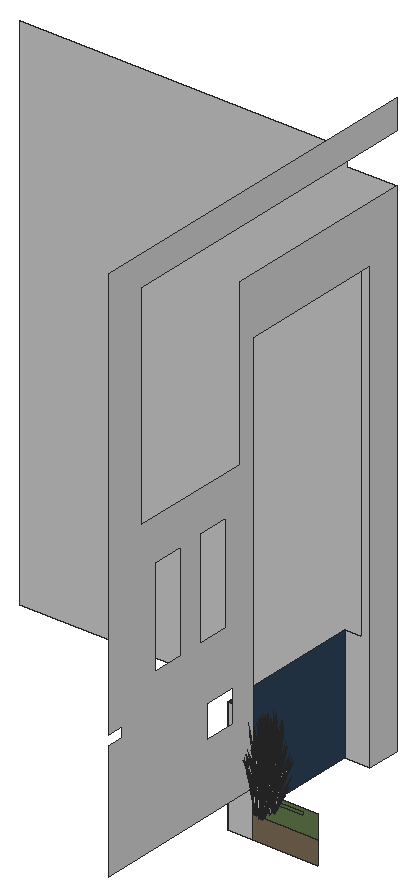
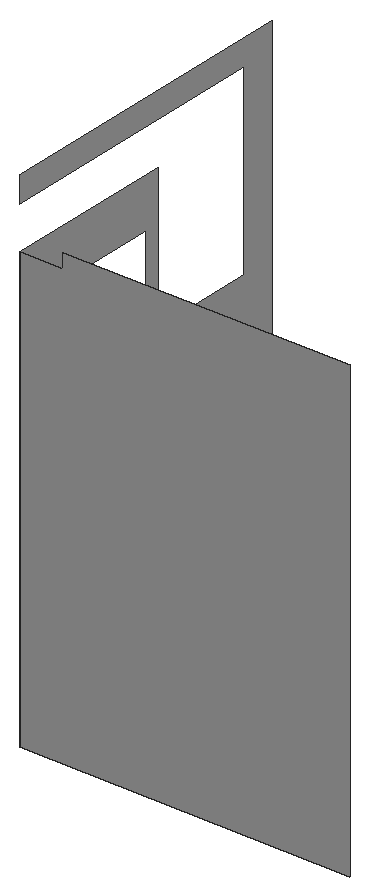
# SketchUp Ruby script. Lengths in inches.
U = 1.inch
M = Sketchup.active_model
def pt(a) = Geom::Point3d.new(a.map { |v| v * U })
def face(e, loops, mat)
  f = e.add_face(loops[0].map { |a| pt(a) })
  loops[1..].each { |l| e.add_face(l.map { |a| pt(a) }).erase! }
  f.material = f.back_material = mat if mat
  f
end
# faces: each face lists its corners as indices into pts; further lists are holes
def faces(e, pts, list, mat = nil) = list.each { |f| face(e, (f[0].is_a?(Array) ? f : [f]).map { |l| l.map { |i| pts[i] } }, mat) }
# xy, xz, yz: faces in a plane at the given z, y or x. An outline is a flat list of corners, or four numbers for a rectangle; further outlines are holes
def ring(l) = l.size == 4 ? [[l[0], l[1]], [l[2], l[1]], [l[2], l[3]], [l[0], l[3]]] : l.each_slice(2).to_a
def flat(e, list, mat, &to3) = list.each { |f| face(e, (f[0].is_a?(Array) ? f : [f]).map { |l| ring(l).map { |u, v| to3.(u, v) } }, mat) }
def xy(e, z, list, mat = nil) = flat(e, list, mat) { |x, y| [x, y, z] }
def xz(e, y, list, mat = nil) = flat(e, list, mat) { |x, z| [x, y, z] }
def yz(e, x, list, mat = nil) = flat(e, list, mat) { |y, z| [x, y, z] }
def lines(e, pts, list) = list.each { |a, b| e.add_line(pt(pts[a]), pt(pts[b])) }
# prism: a flat outline (further loops are holes) pulled along v
def prism(e, loops, v, mat = nil)
  f = face(e, loops, mat); d = Geom::Vector3d.new(v.map { |x| x * U })
  f.pushpull(f.normal.samedirection?(d) ? d.length : -d.length)
end
def box(e, o, s, mat = nil) = prism(e, [[o, [o[0] + s[0], o[1], o[2]], [o[0] + s[0], o[1] + s[1], o[2]], [o[0], o[1] + s[1], o[2]]]], [0, 0, s[2]], mat)
def at(x, y, z, deg = 0) = Geom::Transformation.translation(pt([x, y, z])) * Geom::Transformation.rotation(ORIGIN, Z_AXIS, deg.degrees)
def axes(o, x, y, z) = Geom::Transformation.new([*x, 0, *y, 0, *z, 0, *pt(o).to_a, 1])
def part(name) = M.definitions.add(name)
# library, detail: a bought-in or finely detailed component or shape, given as its bounding box
def library(name, o, s) = part(name).tap { |d| box(d.entities, o, s) }
def detail(e, o, s) = box(e.add_group.entities, o, s)
def put(e, d, t, mat = nil) = e.add_instance(d, t).tap { |i| i.material = mat if mat }
def group(e, t, mat = nil) = e.add_group.tap { |g| g.transformation = t; g.material = mat if mat }.entities
root = M.entities
M.materials.add("Carpet_04_1K").color = [43, 65, 85]
M.materials.add("LightPink_Translucent").color = [144, 107, 117]
M.materials["LightPink_Translucent"].alpha = 0.75
M.materials.add("Plaster_03_1K").color = [121, 105, 83]
M.materials.add("Roofing_02_1K").color = [97, 118, 74]
M.materials.add("[_0053_Ivory_]").color = [200, 200, 200]
c1 = part("blade")
p = [[2.15,0.21,22],[0,0.17,0],[0.09,0.45,0],[2.18,0.31,22],[2.29,0.31,22],[0.38,0.45,0],
  [2.48,0.24,33],[2.49,0.24,33],[2.48,0.22,33]]
faces(c1.entities,p,[[0,1,2,3],[4,5,2,3],[6,3,4,7],[8,0,3,6]])
c2 = part("seeds")
p = [[0.3,-0.1,1.38],[-0.01,-0.03,1.59],[-0.01,-0.03,0.03],[0.14,-0.07,-0.07],[0.29,-0.03,3],[0.15,0.01,3.11]]
faces(c2.entities,p,[[0,1,2,3],[1,0,4,5]],"LightPink_Translucent")
c3 = part("blade with seeds")
put(c3.entities,c1,at(0,0,0))
put(c3.entities,c2,axes([2.4,0.25,30.99],[1.5799,-0.05474,1.17369],[-0.12525,1.92788,0.29478],[-0.07173,-0.02425,1.56792]))
xz(root,365.15,[[659.51,34,695.51,36]],"Roofing_02_1K")
xz(root,371.15,[[653.51,0,701.51,17]],"Plaster_03_1K")
xz(root,371.15,[[653.51,17,701.51,34]],"Roofing_02_1K")
xz(root,371.15,[[635.1,0,653.51,84]],"[_0053_Ivory_]")
xz(root,479.15,[[635.1,0,653.51,0,653.51,330,647.1,330,647.1,84,635.1,84]],"[_0053_Ivory_]")
xz(root,503.15,[[377.51,0,377.51,384,617.51,384,617.51,372,653.51,372,653.51,0]],"[_0053_Ivory_]")
yz(root,635.1,[[371.15,0,479.15,84]],"Carpet_04_1K")
yz(root,653.51,[[[479.15,0,503.15,0,503.15,372,359.15,372,359.15,252,269.15,252,269.15,408,503.15,408,503.15,430,239.15,430,239.15,127,251.15,127,251.15,120,239.15,120,239.15,34,371.15,34,371.15,84,329.15,84,329.15,108,353.15,108,353.15,84,371.15,84,371.15,330,479.15,330],[323.15,150,347.15,222],[281.15,150,305.15,222]]],"[_0053_Ivory_]")
put(root,c3,axes([677.21,343.38,38.33],[-0.16454,0.57202,-0.51099],[-0.56413,-0.19607,-0.3958],[-0.22713,0.05245,0.97773]),"[_0053_Ivory_]")
put(root,c3,axes([680.74,343.13,35.86],[0.36485,0.52782,-0.44739],[-0.55265,0.37168,0.21531],[0.11807,0.06531,1.43643]),"[_0053_Ivory_]")
put(root,c3,axes([683.21,345.36,37.58],[-0.11624,-0.52862,-0.03492],[0.54943,-0.12153,-0.15832],[0.11473,0.03351,0.52218]),"[_0053_Ivory_]")
put(root,c3,axes([678.47,345.83,36.03],[-0.37973,0.63014,0],[-0.6353,-0.35142,-0.51607],[-0.14469,-0.08004,1.63711]),"[_0053_Ivory_]")
put(root,c3,axes([682.35,343.64,36.13],[0,-0.62885,0.49651],[0.67951,0,0],[0,0.14322,1.57504]),"[_0053_Ivory_]")
put(root,c3,axes([680.65,344.11,36.37],[0.65953,-0.03882,0.44739],[0.05964,0.64439,-0.21531],[-0.11807,0.06531,1.43643]),"[_0053_Ivory_]")
put(root,c3,axes([681.06,343.45,36.27],[0.56587,-0.18339,0.1448],[0.19817,0.52368,-0.41347],[0,0.11525,1.26744]),"[_0053_Ivory_]")
put(root,c3,axes([680.06,344.42,35.86],[-0.65953,0.03882,-0.44739],[-0.05964,-0.64439,0.21531],[-0.11807,0.06531,1.43643]),"[_0053_Ivory_]")
put(root,c3,axes([683.16,344.73,36.24],[-0.14627,-0.15466,1.43002],[0.19032,-0.51164,-0.30754],[0.29594,0.06931,0.61141]),"[_0053_Ivory_]")
put(root,c3,axes([680.55,345.29,35.86],[0.61229,0.28233,0],[-0.29468,0.58663,0],[0,0,1.74954]),"[_0053_Ivory_]")
put(root,c3,axes([680.79,345.92,35.85],[-0.37499,-0.63235,-0.05142],[0.6353,-0.35142,0.51607],[-0.15655,0.0602,1.6363]),"[_0053_Ivory_]")
put(root,c3,axes([680.66,344.39,36.27],[0.44871,0.37783,0.1448],[-0.37428,0.42627,-0.41347],[-0.10418,0.05763,1.26744]),"[_0053_Ivory_]")
put(root,c3,axes([677.1875,343.68,37.53],[0.21074,-0.13302,1.71376],[0.17741,0.61464,0.13857],[-0.33083,0.13891,0.73262]),"[_0053_Ivory_]")
put(root,c3,axes([678.49,351.64,37.53],[0.13883,0.2019,1.71376],[-0.64153,0.16998,0.13857],[-0.14499,-0.31697,0.73262]),"[_0053_Ivory_]")
put(root,c3,axes([681.82,345.04,38.63],[0.60713,0.01514,-0.71045],[-0.04078,0.63759,0.08574],[0.25721,0.06729,1.00501]),"[_0053_Ivory_]")
put(root,c3,axes([680.98,351.35,36.24],[-0.17264,0.12729,1.43002],[-0.51703,-0.22279,-0.30754],[0.09584,-0.27707,0.61141]),"[_0053_Ivory_]")
put(root,c3,axes([681.13,345.55,36.13],[0.56842,-0.31443,0.49651],[0.33976,0.56381,0],[-0.12946,0.07161,1.57504]),"[_0053_Ivory_]")
put(root,c3,axes([680.2,351.79,38.63],[-0.28988,-0.51132,-0.71045],[0.59671,-0.28496,0.08574],[-0.06778,-0.24706,1.00501]),"[_0053_Ivory_]")
put(root,c3,axes([680.32,345.06,35.94],[0.26406,0.72244,-0.06012],[-0.7545,0.25315,0],[0.00922,0.02523,1.72173]),"[_0053_Ivory_]")
put(root,c3,axes([678.3125,351.11,36.24],[-0.03678,0.20572,1.43002],[-0.53767,0.17221,-0.30754],[-0.12568,-0.26589,0.61141]),"[_0053_Ivory_]")
put(root,c3,axes([680.62,345.84,35.68],[-0.56663,-0.1556,-0.30978],[0.14267,-0.54795,0.30978],[-0.11423,0.06319,1.38974]),"[_0053_Ivory_]")
put(root,c3,axes([676.53,344.73,36.24],[0.21107,0.05162,1.43002],[0.13604,0.52729,-0.30754],[-0.28671,0.0987,0.61141]),"[_0053_Ivory_]")
put(root,c3,axes([679.7,350.65,35.15],[-0.10187,0.02266,1.76342],[-0.56336,-0.25503,-0.26939],[0.00945,-0.21273,0.30037]),"[_0053_Ivory_]")
put(root,c3,axes([682.81,343.75,36.03],[0.75945,0,0],[0,0.70283,-0.51607],[0,0.16007,1.63711]),"[_0053_Ivory_]")
put(root,c3,axes([682.51,344.11,35.85],[-0.75908,-0.00503,-0.04976],[0,-0.70283,0.49943],[-0.02386,0.16,1.58352]),"[_0053_Ivory_]")
put(root,c3,axes([680.86,343.5,36.32],[0.68399,0.30005,-0.29095],[-0.32934,0.63331,-0.50002],[0.0215,0.15549,1.59708]),"[_0053_Ivory_]")
put(root,c3,axes([676.09,345.83,36.42],[0.25312,-0.28501,1.1486],[0.09988,0.45119,0.84392],[-0.18292,0.08079,0.25299]),"[_0053_Ivory_]")
put(root,c3,axes([682.18,345.3,38.18],[0.34557,0.39372,-0.35414],[-0.39459,0.37271,0.4572],[0.20048,0.05671,0.87481]),"[_0053_Ivory_]")
put(root,c3,axes([682.35,344.21,35.68],[-0.42396,0.39235,-0.30978],[-0.42396,-0.39235,0.30978],[0,0.12637,1.38974]),"[_0053_Ivory_]")
put(root,c3,axes([681.4,352.29,38.63],[0.0158,-0.58168,-0.71045],[0.66548,0.03907,0.08574],[0.07023,-0.24643,1.00501]),"[_0053_Ivory_]")
put(root,c3,axes([680.52,344.25,36.32],[0.07077,0.71755,-0.29095],[-0.73712,0.04339,-0.50002],[-0.1298,0.09558,1.59708]),"[_0053_Ivory_]")
put(root,c3,axes([680.79,343.97,35.86],[-0.29468,0.56664,-0.44739],[-0.61229,-0.27271,0.21531],[0,0.13062,1.43643]),"[_0053_Ivory_]")
put(root,c3,axes([677.04,344.6,38.18],[-0.52868,0.08987,-0.35414],[-0.1396,-0.51376,0.4572],[-0.1515,0.13799,0.87481]),"[_0053_Ivory_]")
put(root,c3,axes([680.25,351.35,38.18],[0.1831,-0.48359,-0.35414],[0.53419,0.14105,0.4572],[-0.04898,-0.1947,0.87481]),"[_0053_Ivory_]")
put(root,c3,axes([680.65,351.99,37.53],[-0.11309,0.21615,1.71376],[-0.47441,-0.44731,0.13857],[0.21402,-0.27879,0.73262]),"[_0053_Ivory_]")
put(root,c3,axes([679.98,351.6875,38.33],[-0.59704,-0.15764,-0.51099],[0.20464,-0.54049,-0.3958],[-0.05475,-0.21761,0.97773]),"[_0053_Ivory_]")
put(root,c3,axes([680.35,350.33,36.42],[0.07791,0.3667,1.1486],[-0.43222,-0.2031,0.84392],[0.04651,-0.18776,0.25299]),"[_0053_Ivory_]")
put(root,c3,axes([681.27,352.1,38.33],[-0.43478,-0.42253,-0.51099],[0.45929,-0.37004,-0.3958],[0.06615,-0.21468,0.97773]),"[_0053_Ivory_]")
put(root,c3,axes([680.08,344.8,35.71],[-0.40909,0.47266,-0.62353],[-0.50819,-0.4286,-0.16365],[-0.16393,0.11791,1.37633]),"[_0053_Ivory_]")
put(root,c3,axes([680.81,345.59,35.98],[0.76036,0.2044,0.30756],[-0.19023,0.7306,-0.36492],[-0.12585,0.09144,1.64885]),"[_0053_Ivory_]")
put(root,c3,axes([680.75,346.09,35.67],[-0.56842,0.31443,-0.49651],[-0.33976,-0.56381,0],[-0.12946,0.07161,1.57504]),"[_0053_Ivory_]")
put(root,c3,axes([682.64,344.22,35.67],[0,0.62885,-0.49651],[-0.67951,0,0],[0,0.14322,1.57504]),"[_0053_Ivory_]")
put(root,c3,axes([680.94,344.29,37.53],[-0.2256,-0.10835,1.71376],[0.46687,-0.45453,0.13857],[0.29098,0.20505,0.73262]),"[_0053_Ivory_]")
put(root,c3,axes([681.78,345.53,36.42],[-0.34197,-0.18082,1.1486],[0.44156,-0.18372,0.84392],[0.1191,0.15563,0.25299]),"[_0053_Ivory_]")
put(root,c3,axes([681.68,351.9375,38.18],[0.41095,-0.33109,-0.35414],[0.38901,0.37805,0.4572],[0.05919,-0.19208,0.87481]),"[_0053_Ivory_]")
put(root,c3,axes([678.125,350.77,36.42],[0.31682,0.21887,1.1486],[-0.4614,0.13157,0.84392],[-0.09872,-0.16821,0.25299]),"[_0053_Ivory_]")
put(root,c3,axes([678.89,351.93,38.63],[-0.51789,-0.30395,-0.71045],[0.36805,-0.53263,0.08574],[-0.18764,-0.18149,1.00501]),"[_0053_Ivory_]")
put(root,c3,axes([678.71,351.53,38.18],[-0.0938,-0.50652,-0.35414],[0.53623,-0.13375,0.4572],[-0.14403,-0.14515,0.87481]),"[_0053_Ivory_]")
put(root,c3,axes([677.96,344.09,37.53],[0.1517,-0.19322,1.71376],[0.38303,0.52154,0.13857],[-0.26271,0.23751,0.73262]),"[_0053_Ivory_]")
put(root,c3,axes([677.48,344.66,38.33],[0.15602,0.5742,-0.51099],[-0.59087,0.10045,-0.3958],[-0.16933,0.15423,0.97773]),"[_0053_Ivory_]")
put(root,c3,axes([681.27,345.99,36.03],[0.37973,0.63014,0],[-0.6353,0.35142,-0.51607],[-0.14469,0.08004,1.63711]),"[_0053_Ivory_]")
put(root,c3,axes([681.87,346.2,35.15],[0.04425,-0.09079,1.76342],[0.55709,-0.26738,-0.26939],[0.16889,0.13839,0.30037]),"[_0053_Ivory_]")
put(root,c3,axes([680.94,343.49,36.5],[-0.01659,-0.59209,1.41272],[0.75089,0.15348,0.59816],[-0.1776,0.32398,1.3335]),"[_0053_Ivory_]")
put(root,c3,axes([681.14,344.14,35.75],[0.2227,0.57576,-0.69212],[-0.64151,0.20736,-0.18165],[0.02462,0.19497,1.52773]),"[_0053_Ivory_]")
put(root,c3,axes([676.76,346.12,35.15],[0.08147,0.06283,1.76342],[0.13814,0.58211,-0.26939],[-0.18056,0.12413,0.30037]),"[_0053_Ivory_]")
put(root,c3,axes([681,345.78,38.33],[0.59932,-0.14948,-0.51099],[0.10484,0.56611,-0.3958],[0.16097,0.16223,0.97773]),"[_0053_Ivory_]")
put(root,c3,axes([677.875,351.43,35.15],[-0.05883,0.08284,1.76342],[-0.59454,0.17861,-0.26939],[-0.14363,-0.16248,0.30037]),"[_0053_Ivory_]")
put(root,c3,axes([678.86,353.71,35.75],[-0.24943,-0.64486,-0.69835],[0.71849,-0.23224,-0.18329],[-0.02757,-0.21836,1.54149]),"[_0053_Ivory_]")
put(root,c3,axes([677.56,352.27,37.53],[0.2256,0.10835,1.71376],[-0.46687,0.45453,0.13857],[-0.29098,-0.20505,0.73262]),"[_0053_Ivory_]")
put(root,c3,axes([682.19,351.74,35.15],[-0.0909,-0.04954,1.76342],[-0.2335,-0.55347,-0.26939],[0.15752,-0.1502,0.30037]),"[_0053_Ivory_]")
put(root,c3,axes([681.83,346.35,36.32],[-0.38947,-0.01972,1.0506],[0.25721,-0.41888,0.58006],[0.15386,0.14882,0.8241]),"[_0053_Ivory_]")
put(root,c3,axes([678.65,351.95,38.33],[-0.59932,0.14948,-0.51099],[-0.10484,-0.56611,-0.3958],[-0.16097,-0.16223,0.97773]),"[_0053_Ivory_]")
put(root,c3,axes([677.84,344.57,37.53],[0.11309,-0.21615,1.71376],[0.47441,0.44731,0.13857],[-0.21402,0.27879,0.73262]),"[_0053_Ivory_]")
put(root,c3,axes([682.1875,353.3,38.63],[0.31725,-0.49618,-0.71045],[0.55593,0.35263,0.08574],[0.18942,-0.17977,1.00501]),"[_0053_Ivory_]")
put(root,c3,axes([678.76,351.86,36.03],[-0.37973,-0.63014,0],[0.6353,-0.35142,-0.51607],[0.14469,-0.08004,1.63711]),"[_0053_Ivory_]")
put(root,c3,axes([682.17,353.07,38.33],[-0.15602,-0.5742,-0.51099],[0.59087,-0.10045,-0.3958],[0.16933,-0.15423,0.97773]),"[_0053_Ivory_]")
put(root,c3,axes([680.56,345.34,36.24],[0.01072,-0.20846,1.43002],[0.51218,-0.23285,-0.30754],[0.15811,0.2495,0.61141]),"[_0053_Ivory_]")
put(root,c3,axes([679.59,351.1,35.78],[-0.4197,0.36076,-0.03893],[-0.38456,-0.39511,-0.17649],[-0.02707,-0.11196,0.58215]),"[_0053_Ivory_]")
put(root,c3,axes([677.97,345.79,38.18],[-0.41095,0.33109,-0.35414],[-0.38901,-0.37805,0.4572],[-0.05919,0.19208,0.87481]),"[_0053_Ivory_]")
put(root,c3,axes([678.24,347.07,36.42],[-0.01572,-0.37392,1.1486],[0.39276,0.26669,0.84392],[-0.07724,0.17822,0.25299]),"[_0053_Ivory_]")
put(root,c3,axes([680.13,355.37,36.98],[0.52485,0.25358,1.51261],[-0.51417,0.54629,0.59816],[-0.23031,-0.32378,1.26806]),"[_0053_Ivory_]")
put(root,c3,axes([679.27,346.18,35.15],[0.09829,-0.03422,1.76342],[0.59126,0.18834,-0.26939],[0.01729,0.21228,0.30037]),"[_0053_Ivory_]")
put(root,c3,axes([677.39,353.62,35.67],[0,-0.62885,-0.49651],[0.67951,0,0],[0,-0.14322,1.57504]),"[_0053_Ivory_]")
put(root,c3,axes([679.27,351.76,35.67],[0.56842,-0.31443,-0.49651],[0.33976,0.56381,0],[0.12946,-0.07161,1.57504]),"[_0053_Ivory_]")
put(root,c3,axes([682.65,352.84,36.24],[-0.21697,-0.01863,1.43002],[-0.22228,-0.49966,-0.30754],[0.26655,-0.14135,0.61141]),"[_0053_Ivory_]")
put(root,c3,axes([678.38,345.63,38.66],[0.43478,0.42253,-0.5672],[-0.45929,0.37004,-0.43934],[-0.06615,0.21468,1.08528]),"[_0053_Ivory_]")
put(root,c3,axes([677.91,346.27,36.48],[0.55175,-0.11136,0.06507],[0.12684,0.44864,-0.86304],[-0.03498,0.22711,0.7736]),"[_0053_Ivory_]")
put(root,c3,axes([679.95,353.05,35.71],[0.40909,-0.47266,-0.62353],[0.50819,0.4286,-0.16365],[0.16393,-0.11791,1.37633]),"[_0053_Ivory_]")
put(root,c3,axes([679.67,346.04,38.33],[0.59704,0.15764,-0.51099],[-0.20464,0.54049,-0.3958],[0.05475,0.21761,0.97773]),"[_0053_Ivory_]")
put(root,c3,axes([680.01,344.92,37.53],[-0.13883,-0.2019,1.71376],[0.64153,-0.16998,0.13857],[0.14499,0.31697,0.73262]),"[_0053_Ivory_]")
put(root,c3,axes([682.9,351.93,36.42],[-0.2023,0.32011,1.1486],[-0.17388,-0.43009,0.84392],[0.16708,-0.10777,0.25299]),"[_0053_Ivory_]")
put(root,c3,axes([679.4,346.37,38.18],[-0.1831,0.48359,-0.35414],[-0.53419,-0.14105,0.4572],[0.04898,0.1947,0.87481]),"[_0053_Ivory_]")
put(root,c3,axes([682.61,353.13,38.18],[0.52868,-0.08987,-0.35414],[0.1396,0.51376,0.4572],[0.1515,-0.13799,0.87481]),"[_0053_Ivory_]")
put(root,c3,axes([678.25,345.4375,38.99],[-0.0158,0.58168,-0.7886],[-0.66548,-0.03907,0.09517],[-0.07023,0.24643,1.11556]),"[_0053_Ivory_]")
put(root,c3,axes([679.24,353.875,35.86],[0.29468,-0.56664,-0.44739],[0.61229,0.27271,0.21531],[0,-0.13062,1.43643]),"[_0053_Ivory_]")
put(root,c3,axes([677.47,352.42,38.18],[-0.34557,-0.39372,-0.35414],[0.39459,-0.37271,0.4572],[-0.20048,-0.05671,0.87481]),"[_0053_Ivory_]")
put(root,c3,axes([679.5,353.6,36.32],[-0.07077,-0.71755,-0.29095],[0.73712,-0.04339,-0.50002],[0.1298,-0.09558,1.59708]),"[_0053_Ivory_]")
put(root,c3,axes([677.68,353.63,35.68],[0.42396,-0.39235,-0.30978],[0.42396,0.39235,0.30978],[0,-0.12637,1.38974]),"[_0053_Ivory_]")
put(root,c3,axes([678.88,345.02,37.53],[-0.01487,-0.24136,1.71376],[0.64429,0.16012,0.13857],[-0.03985,0.34396,0.73262]),"[_0053_Ivory_]")
put(root,c3,axes([677.51,351.75,35.78],[-0.1752,0.51349,-0.03893],[-0.53924,-0.15795,-0.17649],[-0.08187,-0.08399,0.58215]),"[_0053_Ivory_]")
put(root,c3,axes([679.16,354.35,36.32],[-0.68399,-0.30005,-0.29095],[0.32934,-0.63331,-0.50002],[-0.0215,-0.15549,1.59708]),"[_0053_Ivory_]")
put(root,c3,axes([677.22,354.1,36.03],[-0.75945,0,0],[0,-0.70283,-0.51607],[0,-0.16007,1.63711]),"[_0053_Ivory_]")
put(root,c3,axes([677.35,352.84,36.24],[0.11858,0.17508,1.43002],[-0.27325,0.4759,-0.30754],[-0.28057,-0.11375,0.61141]),"[_0053_Ivory_]")
put(root,c3,axes([679.41,352.01,35.68],[0.56663,0.1556,-0.30978],[-0.14267,0.54795,0.30978],[0.11423,-0.06319,1.38974]),"[_0053_Ivory_]")
put(root,c3,axes([679.46,345.9375,38.63],[0.28988,0.51132,-0.71045],[-0.59671,0.28496,0.08574],[0.06778,0.24706,1.00501]),"[_0053_Ivory_]")
put(root,c3,axes([677.83,352.69,38.63],[-0.60713,-0.01514,-0.71045],[0.04078,-0.63759,0.08574],[-0.25721,-0.06729,1.00501]),"[_0053_Ivory_]")
put(root,c3,axes([677.78,346.74,36.24],[0.19166,-0.0992,1.43002],[0.4732,0.29912,-0.30754],[-0.14084,0.25882,0.61141]),"[_0053_Ivory_]")
put(root,c3,axes([677.8,353.91,35.98],[-0.56493,0.5287,0.30756],[-0.56528,-0.52313,-0.36492],[-0.01973,-0.15014,1.64885]),"[_0053_Ivory_]")
put(root,c3,axes([679.6,354.16,36.09],[0.68433,0.30479,0.24065],[-0.32934,0.63331,0.50002],[0,-0.14599,1.60543]),"[_0053_Ivory_]")
put(root,c3,axes([678.03,346.26,37.02],[0.01334,-0.32463,1.54345],[0.60018,0.17147,0.21329],[-0.052,0.34598,0.72882]),"[_0053_Ivory_]")
put(root,c3,axes([679.33,355.01,36.09],[0.16098,-0.74515,-0.23429],[0.76326,0.12989,0.51271],[-0.13337,-0.1029,1.5644]),"[_0053_Ivory_]")
put(root,c3,axes([677.63,352.8125,38.33],[-0.44101,0.41656,-0.51099],[-0.38623,-0.44004,-0.3958],[-0.22407,-0.06338,0.97773]),"[_0053_Ivory_]")
put(root,c3,axes([676.64,353.37,36.42],[0.38775,-0.045,1.1486],[-0.24596,0.39648,0.84392],[-0.19161,-0.05948,0.25299]),"[_0053_Ivory_]")
put(root,c3,axes([679.38,353.73,36.37],[-0.65953,0.03882,0.44739],[-0.05964,-0.64439,-0.21531],[0.11807,-0.06531,1.43643]),"[_0053_Ivory_]")
put(root,c3,axes([677.68,354.2,36.13],[0,0.62885,0.49651],[-0.67951,0,0],[0,-0.14322,1.57504]),"[_0053_Ivory_]")
put(root,c3,axes([682.45,354.34,38.33],[0.16454,-0.57202,-0.51099],[0.56413,0.19607,-0.3958],[0.22713,-0.05245,0.97773]),"[_0053_Ivory_]")
put(root,c3,axes([681.55,352.01,36.03],[0.37973,-0.63014,0],[0.6353,0.35142,-0.51607],[0.14469,0.08004,1.63711]),"[_0053_Ivory_]")
put(root,c3,axes([677.08,353.26,37.53],[0.25192,-0.01424,1.71376],[-0.16712,0.61729,0.13857],[-0.35901,-0.03818,0.73262]),"[_0053_Ivory_]")
put(root,c3,axes([679.28,354.71,35.86],[-0.36485,-0.52782,-0.44739],[0.55265,-0.37168,0.21531],[-0.11807,-0.06531,1.43643]),"[_0053_Ivory_]")
put(root,c3,axes([679.36,353.97,36.01],[0.26406,0.70318,0.45755],[-0.7545,0.24452,0.17955],[0.00922,-0.12921,1.58856]),"[_0053_Ivory_]")
put(root,c3,axes([683.05,354.5,35.64],[-0.39118,0.07547,1.41583],[-0.06226,-0.6007,0.08104],[0.27398,-0.09092,0.80566]),"[_0053_Ivory_]")
put(root,c3,axes([683.76,353.97,35.91],[-0.37654,-0.40212,-0.06488],[0.4124,-0.36845,-0.29416],[0.11685,-0.02594,0.97024]),"[_0053_Ivory_]")
put(root,c3,axes([679.22,354.52,36.37],[-0.29468,0.56664,0.44739],[-0.61229,-0.27271,-0.21531],[0,-0.13062,1.43643]),"[_0053_Ivory_]")
put(root,c3,axes([680.31,354.02,35.86],[0,-0.72763,0],[0.75945,0,0],[0,0,1.79456]),"[_0053_Ivory_]")
put(root,c3,axes([681.23,352.34,36.13],[-0.56842,-0.31443,0.49651],[0.33976,-0.56381,0],[0.12946,0.07161,1.57504]),"[_0053_Ivory_]")
put(root,c3,axes([682.34,354.55,38.63],[0.53369,-0.27773,-0.71045],[0.29743,0.5717,0.08574],[0.25786,-0.06494,1.00501]),"[_0053_Ivory_]")
put(root,c3,axes([678.95,354.91,35.71],[-0.63179,-0.1031,-0.62353],[0.13332,-0.63596,-0.16365],[-0.18854,-0.07706,1.37633]),"[_0053_Ivory_]")
put(root,c3,axes([679.95,353.57,36.01],[-0.50358,0.57069,0.45755],[-0.59827,-0.50377,0.17955],[0.1214,-0.05695,1.58856]),"[_0053_Ivory_]")
put(root,c3,axes([680.5,354.59,35.95],[-0.56493,-0.54126,-0.06131],[0.56528,-0.54159,0],[-0.01973,-0.0189,1.75571]),"[_0053_Ivory_]")
put(root,c3,axes([679.07,352.625,36.13],[-0.17545,0.62497,0.17642],[-0.64204,-0.17686,0.35086],[0.11091,-0.00304,1.60407]),"[_0053_Ivory_]")
put(root,c3,axes([678.81,353.13,35.25],[-0.59782,0.25177,1.28929],[-0.19028,-0.72239,0.50096],[0.36709,0.01202,1.46642]),"[_0053_Ivory_]")
put(root,c3,axes([680.41,353.32,36.27],[0.11717,-0.56122,0.1448],[0.57245,0.09742,-0.41347],[0.10418,0.05763,1.26744]),"[_0053_Ivory_]")
put(root,c3,axes([679.42,354.65,36.01],[0.76764,0.13249,0.45755],[-0.15622,0.74829,0.17955],[-0.11218,-0.07226,1.58856]),"[_0053_Ivory_]")
put(root,c3,axes([683.48,354.11,35.15],[-0.03174,-0.09547,1.76342],[0.22015,-0.55846,-0.26939],[0.22208,-0.00803,0.30037]),"[_0053_Ivory_]")
put(root,c3,axes([676.92,354.01,35.15],[0.0154,0.09911,1.76342],[-0.31051,0.51756,-0.26939],[-0.22056,-0.02609,0.30037]),"[_0053_Ivory_]")
put(root,c3,axes([680.17,353.47,36.37],[-0.36485,-0.52782,0.44739],[0.55265,-0.37168,-0.21531],[0.11807,0.06531,1.43643]),"[_0053_Ivory_]")
put(root,c3,axes([678.28,355.88,35.68],[-0.14267,-0.54795,-0.30978],[0.56663,-0.1556,0.30978],[-0.11423,-0.06319,1.38974]),"[_0053_Ivory_]")
put(root,c3,axes([679.01,355.85,36.13],[0.65264,-0.16691,0.17642],[0.16115,0.62115,0.35086],[-0.05821,-0.0905,1.60407]),"[_0053_Ivory_]")
put(root,c3,axes([680.35,353.5,36.32],[0.61322,-0.4175,-0.29095],[0.40778,0.58992,-0.50002],[0.1513,0.05991,1.59708]),"[_0053_Ivory_]")
put(root,c3,axes([682.79,354.6,38.18],[0.50475,0.17543,-0.35414],[-0.14722,0.5118,0.4572],[0.20322,-0.04693,0.87481]),"[_0053_Ivory_]")
put(root,c3,axes([678.125,356.12,35.67],[-0.56842,-0.31443,-0.49651],[0.33976,-0.56381,0],[-0.12946,-0.07161,1.57504]),"[_0053_Ivory_]")
put(root,c3,axes([681.9,352.39,35.67],[0.56842,0.31443,-0.49651],[-0.33976,0.56381,0],[0.12946,0.07161,1.57504]),"[_0053_Ivory_]")
put(root,c3,axes([676.86,353.79,38.18],[-0.50475,-0.17543,-0.35414],[0.14722,-0.5118,0.4572],[-0.20322,0.04693,0.87481]),"[_0053_Ivory_]")
put(root,c3,axes([680.82,354.1875,35.86],[0.67951,0,0],[0,0.65103,0],[0,0,1.78407]),"[_0053_Ivory_]")
put(root,c3,axes([679.67,355.01,36.32],[-0.61322,0.4175,-0.29095],[-0.40778,-0.58992,-0.50002],[-0.1513,-0.05991,1.59708]),"[_0053_Ivory_]")
put(root,c3,axes([681.01,352.66,36.13],[-0.65264,0.16691,0.17642],[-0.16115,-0.62115,0.35086],[0.05821,0.0905,1.60407]),"[_0053_Ivory_]")
put(root,c3,axes([681.42,353.97,37.53],[-0.25192,0.01424,1.71376],[0.16712,-0.61729,0.13857],[0.35901,0.03818,0.73262]),"[_0053_Ivory_]")
put(root,c3,axes([681.74,352.63,35.68],[0.14267,0.54795,-0.30978],[-0.56663,0.1556,0.30978],[0.11423,0.06319,1.38974]),"[_0053_Ivory_]")
put(root,c3,axes([680.6,353.86,36.03],[-0.76764,-0.13249,0.49198],[0.15622,-0.74829,0.19306],[0.11218,0.07226,1.70813]),"[_0053_Ivory_]")
put(root,c3,axes([679.99,355.7,35.86],[-0.19817,-0.54216,0],[0.56587,-0.18986,0],[0,0,1.54371]),"[_0053_Ivory_]")
put(root,c3,axes([679.61,355.1875,36.27],[-0.11717,0.56122,0.1448],[-0.57245,-0.09742,-0.41347],[-0.10418,-0.05763,1.26744]),"[_0053_Ivory_]")
put(root,c3,axes([680.73,355.63,35.84],[0.63764,-0.21337,-0.19198],[0.22406,0.61462,0.00008],[0.07038,-0.02358,1.73897]),"[_0053_Ivory_]")
put(root,c3,axes([680.95,355.88,36.13],[0.17545,-0.62497,0.17642],[0.64204,0.17686,0.35086],[-0.11091,0.00304,1.60407]),"[_0053_Ivory_]")
put(root,c3,axes([680.81,354.47,35.87],[0.42396,0.40619,0],[-0.42396,0.40619,0],[0,0,1.69266]),"[_0053_Ivory_]")
put(root,c3,axes([678.4,353.7,37],[0.17264,-0.09097,1.77064],[0.05953,0.63516,0.13857],[-0.37394,0.08428,0.63284]),"[_0053_Ivory_]")
put(root,c3,axes([681.95,354.29,36.13],[-0.47719,-0.45806,0.17642],[0.48088,-0.44429,0.35086],[-0.0527,0.09355,1.60407]),"[_0053_Ivory_]")
put(root,c3,axes([681.07,353.6,35.71],[0.63179,0.1031,-0.62353],[-0.13332,0.63596,-0.16365],[0.18854,0.07706,1.37633]),"[_0053_Ivory_]")
put(root,c3,axes([683.86,354.71,36.42],[-0.37526,0.10382,1.1486],[0.17664,-0.42906,0.84392],[0.19907,0.02936,0.25299]),"[_0053_Ivory_]")
put(root,c3,axes([679.85,355.95,35.85],[-0.61229,-0.28233,0],[0.29468,-0.58663,0],[0,0,1.62707]),"[_0053_Ivory_]")
put(root,c3,axes([680.36,355.2,36.12],[-0.59306,-0.50614,-0.25192],[0.49904,-0.56836,0.5513],[-0.1597,0.05921,1.68216]),"[_0053_Ivory_]")
put(root,c3,axes([678.8,356.17,36.13],[0.56842,0.31443,0.49651],[-0.33976,0.56381,0],[-0.12946,-0.07161,1.57504]),"[_0053_Ivory_]")
put(root,c3,axes([680.8,353.99,36.37],[0.29468,-0.56664,0.44739],[0.61229,0.27271,-0.21531],[0,0.13062,1.43643]),"[_0053_Ivory_]")
put(root,c3,axes([680.6875,354.32,35.95],[0,0.72727,-0.05637],[-0.75945,0,0],[0,0.02286,1.79368]),"[_0053_Ivory_]")
put(root,c3,axes([677.21,354.05,38.33],[-0.16454,0.57202,-0.51099],[-0.56413,-0.19607,-0.3958],[-0.22713,0.05245,0.97773]),"[_0053_Ivory_]")
put(root,c3,axes([680.74,353.8,35.86],[0.36485,0.52782,-0.44739],[-0.55265,0.37168,0.21531],[0.11807,0.06531,1.43643]),"[_0053_Ivory_]")
put(root,c3,axes([683.21,356.03,37.58],[-0.11624,-0.52862,-0.03492],[0.54943,-0.12153,-0.15832],[0.11473,0.03351,0.52218]),"[_0053_Ivory_]")
put(root,c3,axes([678.47,356.5,36.03],[-0.37973,0.63014,0],[-0.6353,-0.35142,-0.51607],[-0.14469,-0.08004,1.63711]),"[_0053_Ivory_]")
put(root,c3,axes([682.35,354.31,36.13],[0,-0.62885,0.49651],[0.67951,0,0],[0,0.14322,1.57504]),"[_0053_Ivory_]")
put(root,c3,axes([680.65,354.78,36.37],[0.65953,-0.03882,0.44739],[0.05964,0.64439,-0.21531],[-0.11807,0.06531,1.43643]),"[_0053_Ivory_]")
put(root,c3,axes([681.06,354.12,36.27],[0.56587,-0.18339,0.1448],[0.19817,0.52368,-0.41347],[0,0.11525,1.26744]),"[_0053_Ivory_]")
put(root,c3,axes([680.06,355.09,35.86],[-0.65953,0.03882,-0.44739],[-0.05964,-0.64439,0.21531],[-0.11807,0.06531,1.43643]),"[_0053_Ivory_]")
put(root,c3,axes([683.16,355.4,36.24],[-0.14627,-0.15466,1.43002],[0.19032,-0.51164,-0.30754],[0.29594,0.06931,0.61141]),"[_0053_Ivory_]")
put(root,c3,axes([680.55,355.96,35.86],[0.61229,0.28233,0],[-0.29468,0.58663,0],[0,0,1.74954]),"[_0053_Ivory_]")
put(root,c3,axes([680.79,356.58,35.85],[-0.37499,-0.63235,-0.05142],[0.6353,-0.35142,0.51607],[-0.15655,0.0602,1.6363]),"[_0053_Ivory_]")
put(root,c3,axes([680.66,355.05,36.27],[0.44871,0.37783,0.1448],[-0.37428,0.42627,-0.41347],[-0.10418,0.05763,1.26744]),"[_0053_Ivory_]")
put(root,c3,axes([677.1875,354.35,37.53],[0.21074,-0.13302,1.71376],[0.17741,0.61464,0.13857],[-0.33083,0.13891,0.73262]),"[_0053_Ivory_]")
put(root,c3,axes([681.82,355.71,38.63],[0.60713,0.01514,-0.71045],[-0.04078,0.63759,0.08574],[0.25721,0.06729,1.00501]),"[_0053_Ivory_]")
put(root,c3,axes([681.13,356.22,36.13],[0.56842,-0.31443,0.49651],[0.33976,0.56381,0],[-0.12946,0.07161,1.57504]),"[_0053_Ivory_]")
put(root,c3,axes([680.32,355.72,35.94],[0.26406,0.72244,-0.06012],[-0.7545,0.25315,0],[0.00922,0.02523,1.72173]),"[_0053_Ivory_]")
put(root,c3,axes([680.62,356.5,35.68],[-0.56663,-0.1556,-0.30978],[0.14267,-0.54795,0.30978],[-0.11423,0.06319,1.38974]),"[_0053_Ivory_]")
put(root,c3,axes([676.53,355.39,36.24],[0.21107,0.05162,1.43002],[0.13604,0.52729,-0.30754],[-0.28671,0.0987,0.61141]),"[_0053_Ivory_]")
put(root,c3,axes([682.81,354.41,36.03],[0.75945,0,0],[0,0.70283,-0.51607],[0,0.16007,1.63711]),"[_0053_Ivory_]")
put(root,c3,axes([682.51,354.78,35.85],[-0.75908,-0.00503,-0.04976],[0,-0.70283,0.49943],[-0.02386,0.16,1.58352]),"[_0053_Ivory_]")
put(root,c3,axes([680.86,354.16,36.32],[0.68399,0.30005,-0.29095],[-0.32934,0.63331,-0.50002],[0.0215,0.15549,1.59708]),"[_0053_Ivory_]")
put(root,c3,axes([676.09,356.5,36.42],[0.25312,-0.28501,1.1486],[0.09988,0.45119,0.84392],[-0.18292,0.08079,0.25299]),"[_0053_Ivory_]")
put(root,c3,axes([682.18,355.97,38.18],[0.34557,0.39372,-0.35414],[-0.39459,0.37271,0.4572],[0.20048,0.05671,0.87481]),"[_0053_Ivory_]")
put(root,c3,axes([682.35,354.88,35.68],[-0.42396,0.39235,-0.30978],[-0.42396,-0.39235,0.30978],[0,0.12637,1.38974]),"[_0053_Ivory_]")
put(root,c3,axes([680.52,354.92,36.32],[0.07077,0.71755,-0.29095],[-0.73712,0.04339,-0.50002],[-0.1298,0.09558,1.59708]),"[_0053_Ivory_]")
put(root,c3,axes([680.79,354.63,35.86],[-0.29468,0.56664,-0.44739],[-0.61229,-0.27271,0.21531],[0,0.13062,1.43643]),"[_0053_Ivory_]")
put(root,c3,axes([677.04,355.26,38.18],[-0.52868,0.08987,-0.35414],[-0.1396,-0.51376,0.4572],[-0.1515,0.13799,0.87481]),"[_0053_Ivory_]")
put(root,c3,axes([680.08,355.46,35.71],[-0.40909,0.47266,-0.62353],[-0.50819,-0.4286,-0.16365],[-0.16393,0.11791,1.37633]),"[_0053_Ivory_]")
put(root,c3,axes([680.81,356.26,35.98],[0.76036,0.2044,0.30756],[-0.19023,0.7306,-0.36492],[-0.12585,0.09144,1.64885]),"[_0053_Ivory_]")
put(root,c3,axes([680.75,356.75,35.67],[-0.56842,0.31443,-0.49651],[-0.33976,-0.56381,0],[-0.12946,0.07161,1.57504]),"[_0053_Ivory_]")
put(root,c3,axes([682.64,354.89,35.67],[0,0.62885,-0.49651],[-0.67951,0,0],[0,0.14322,1.57504]),"[_0053_Ivory_]")
put(root,c3,axes([680.94,354.96,37.53],[-0.2256,-0.10835,1.71376],[0.46687,-0.45453,0.13857],[0.29098,0.20505,0.73262]),"[_0053_Ivory_]")
put(root,c3,axes([681.78,356.2,36.42],[-0.34197,-0.18082,1.1486],[0.44156,-0.18372,0.84392],[0.1191,0.15563,0.25299]),"[_0053_Ivory_]")
put(root,c3,axes([677.96,354.76,37.53],[0.1517,-0.19322,1.71376],[0.38303,0.52154,0.13857],[-0.26271,0.23751,0.73262]),"[_0053_Ivory_]")
put(root,c3,axes([677.48,355.33,38.33],[0.15602,0.5742,-0.51099],[-0.59087,0.10045,-0.3958],[-0.16933,0.15423,0.97773]),"[_0053_Ivory_]")
put(root,c3,axes([681.27,356.66,36.03],[0.37973,0.63014,0],[-0.6353,0.35142,-0.51607],[-0.14469,0.08004,1.63711]),"[_0053_Ivory_]")
put(root,c3,axes([681.87,356.87,35.15],[0.04425,-0.09079,1.76342],[0.55709,-0.26738,-0.26939],[0.16889,0.13839,0.30037]),"[_0053_Ivory_]")
put(root,c3,axes([680.94,354.16,36.5],[-0.01659,-0.59209,1.41272],[0.75089,0.15348,0.59816],[-0.1776,0.32398,1.3335]),"[_0053_Ivory_]")
put(root,c3,axes([681.14,354.81,35.75],[0.2227,0.57576,-0.69212],[-0.64151,0.20736,-0.18165],[0.02462,0.19497,1.52773]),"[_0053_Ivory_]")
put(root,c3,axes([676.76,356.79,35.15],[0.08147,0.06283,1.76342],[0.13814,0.58211,-0.26939],[-0.18056,0.12413,0.30037]),"[_0053_Ivory_]")
put(root,c3,axes([681,356.44,38.33],[0.59932,-0.14948,-0.51099],[0.10484,0.56611,-0.3958],[0.16097,0.16223,0.97773]),"[_0053_Ivory_]")
put(root,c3,axes([681.83,357.02,36.32],[-0.38947,-0.01972,1.0506],[0.25721,-0.41888,0.58006],[0.15386,0.14882,0.8241]),"[_0053_Ivory_]")
put(root,c3,axes([677.84,355.24,37.53],[0.11309,-0.21615,1.71376],[0.47441,0.44731,0.13857],[-0.21402,0.27879,0.73262]),"[_0053_Ivory_]")
put(root,c3,axes([680.56,356,36.24],[0.01072,-0.20846,1.43002],[0.51218,-0.23285,-0.30754],[0.15811,0.2495,0.61141]),"[_0053_Ivory_]")
put(root,c3,axes([677.97,356.45,38.18],[-0.41095,0.33109,-0.35414],[-0.38901,-0.37805,0.4572],[-0.05919,0.19208,0.87481]),"[_0053_Ivory_]")
put(root,c3,axes([678.24,357.74,36.42],[-0.01572,-0.37392,1.1486],[0.39276,0.26669,0.84392],[-0.07724,0.17822,0.25299]),"[_0053_Ivory_]")
put(root,c3,axes([679.27,356.85,35.15],[0.09829,-0.03422,1.76342],[0.59126,0.18834,-0.26939],[0.01729,0.21228,0.30037]),"[_0053_Ivory_]")
put(root,c3,axes([678.38,356.3,38.66],[0.43478,0.42253,-0.5672],[-0.45929,0.37004,-0.43934],[-0.06615,0.21468,1.08528]),"[_0053_Ivory_]")
put(root,c3,axes([677.91,356.93,36.48],[0.55175,-0.11136,0.06507],[0.12684,0.44864,-0.86304],[-0.03498,0.22711,0.7736]),"[_0053_Ivory_]")
put(root,c3,axes([679.67,356.71,38.33],[0.59704,0.15764,-0.51099],[-0.20464,0.54049,-0.3958],[0.05475,0.21761,0.97773]),"[_0053_Ivory_]")
put(root,c3,axes([680.01,355.59,37.53],[-0.13883,-0.2019,1.71376],[0.64153,-0.16998,0.13857],[0.14499,0.31697,0.73262]),"[_0053_Ivory_]")
put(root,c3,axes([679.4,357.04,38.18],[-0.1831,0.48359,-0.35414],[-0.53419,-0.14105,0.4572],[0.04898,0.1947,0.87481]),"[_0053_Ivory_]")
put(root,c3,axes([678.25,356.1,38.99],[-0.0158,0.58168,-0.7886],[-0.66548,-0.03907,0.09517],[-0.07023,0.24643,1.11556]),"[_0053_Ivory_]")
put(root,c3,axes([678.88,355.69,37.53],[-0.01487,-0.24136,1.71376],[0.64429,0.16012,0.13857],[-0.03985,0.34396,0.73262]),"[_0053_Ivory_]")
put(root,c3,axes([679.46,356.6,38.63],[0.28988,0.51132,-0.71045],[-0.59671,0.28496,0.08574],[0.06778,0.24706,1.00501]),"[_0053_Ivory_]")
put(root,c3,axes([677.78,357.41,36.24],[0.19166,-0.0992,1.43002],[0.4732,0.29912,-0.30754],[-0.14084,0.25882,0.61141]),"[_0053_Ivory_]")
put(root,c3,axes([678.03,356.92,37.02],[0.01334,-0.32463,1.54345],[0.60018,0.17147,0.21329],[-0.052,0.34598,0.72882]),"[_0053_Ivory_]")
